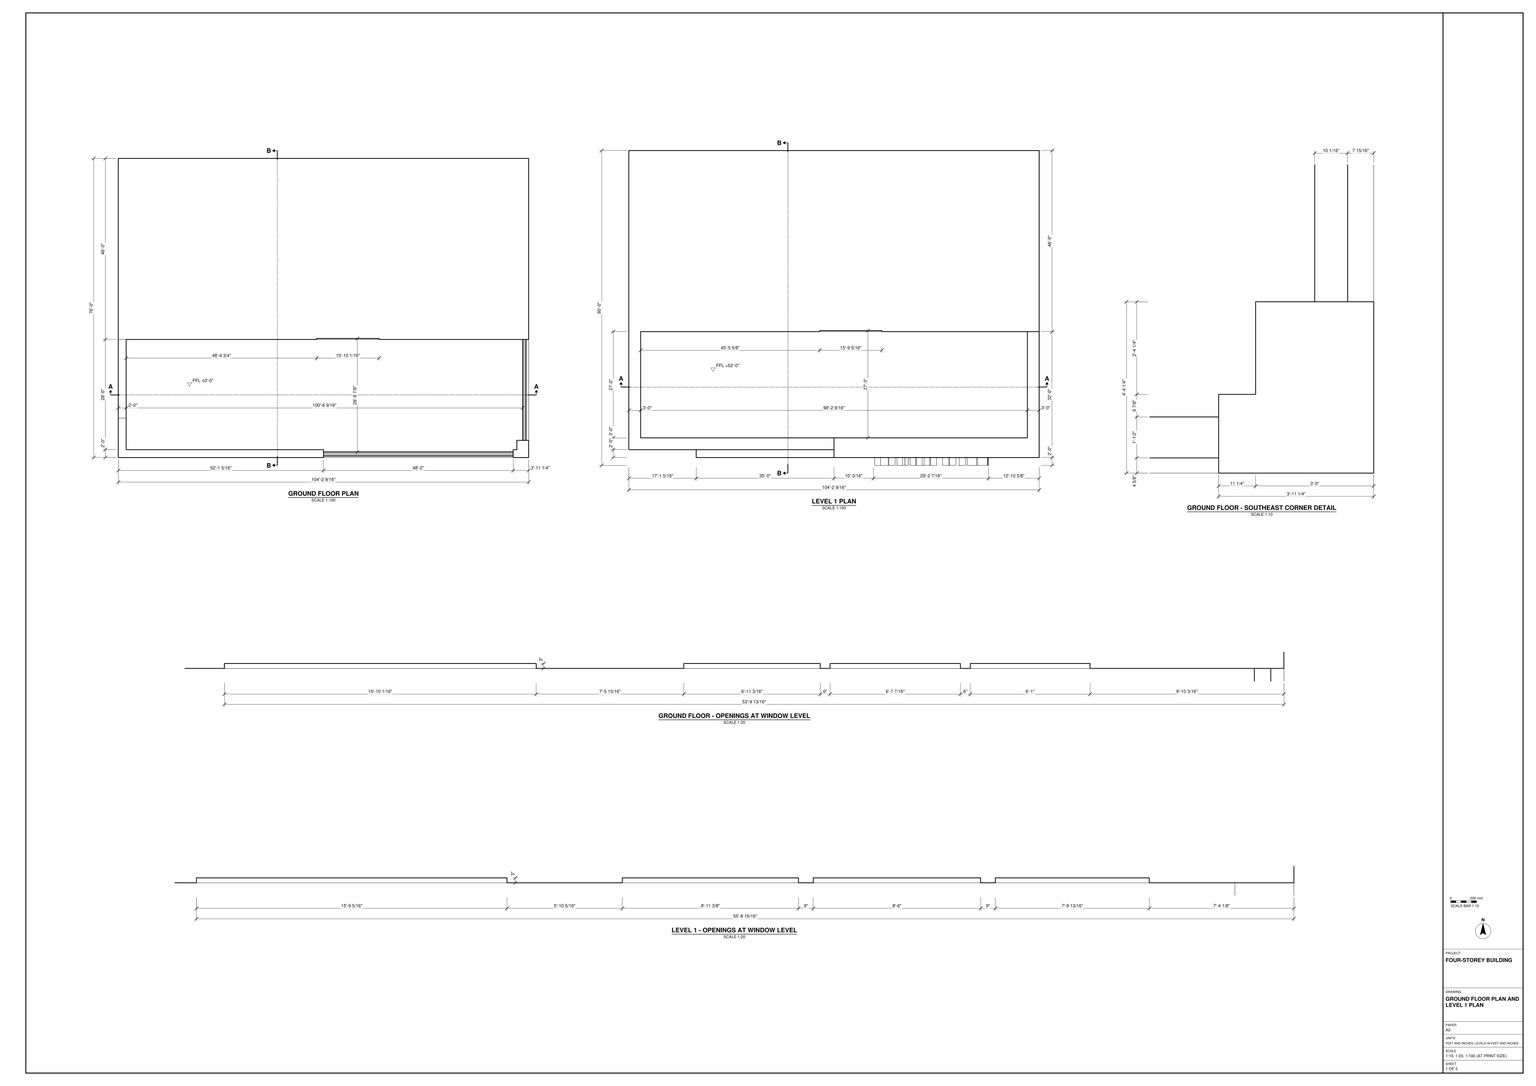
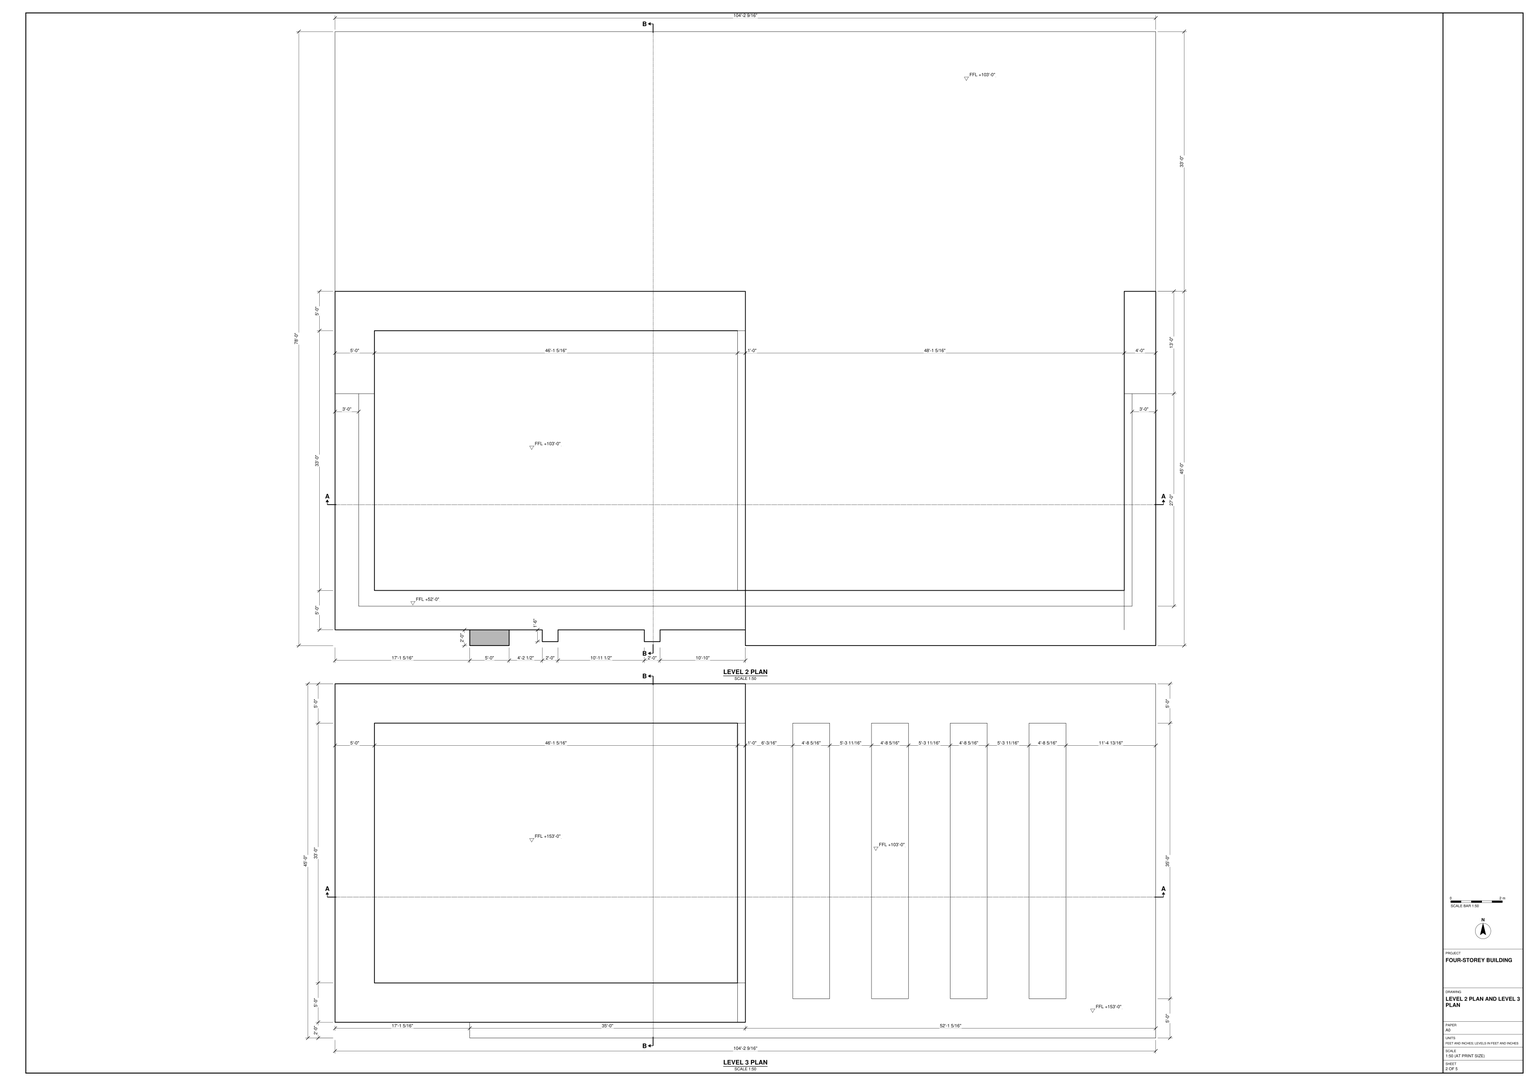
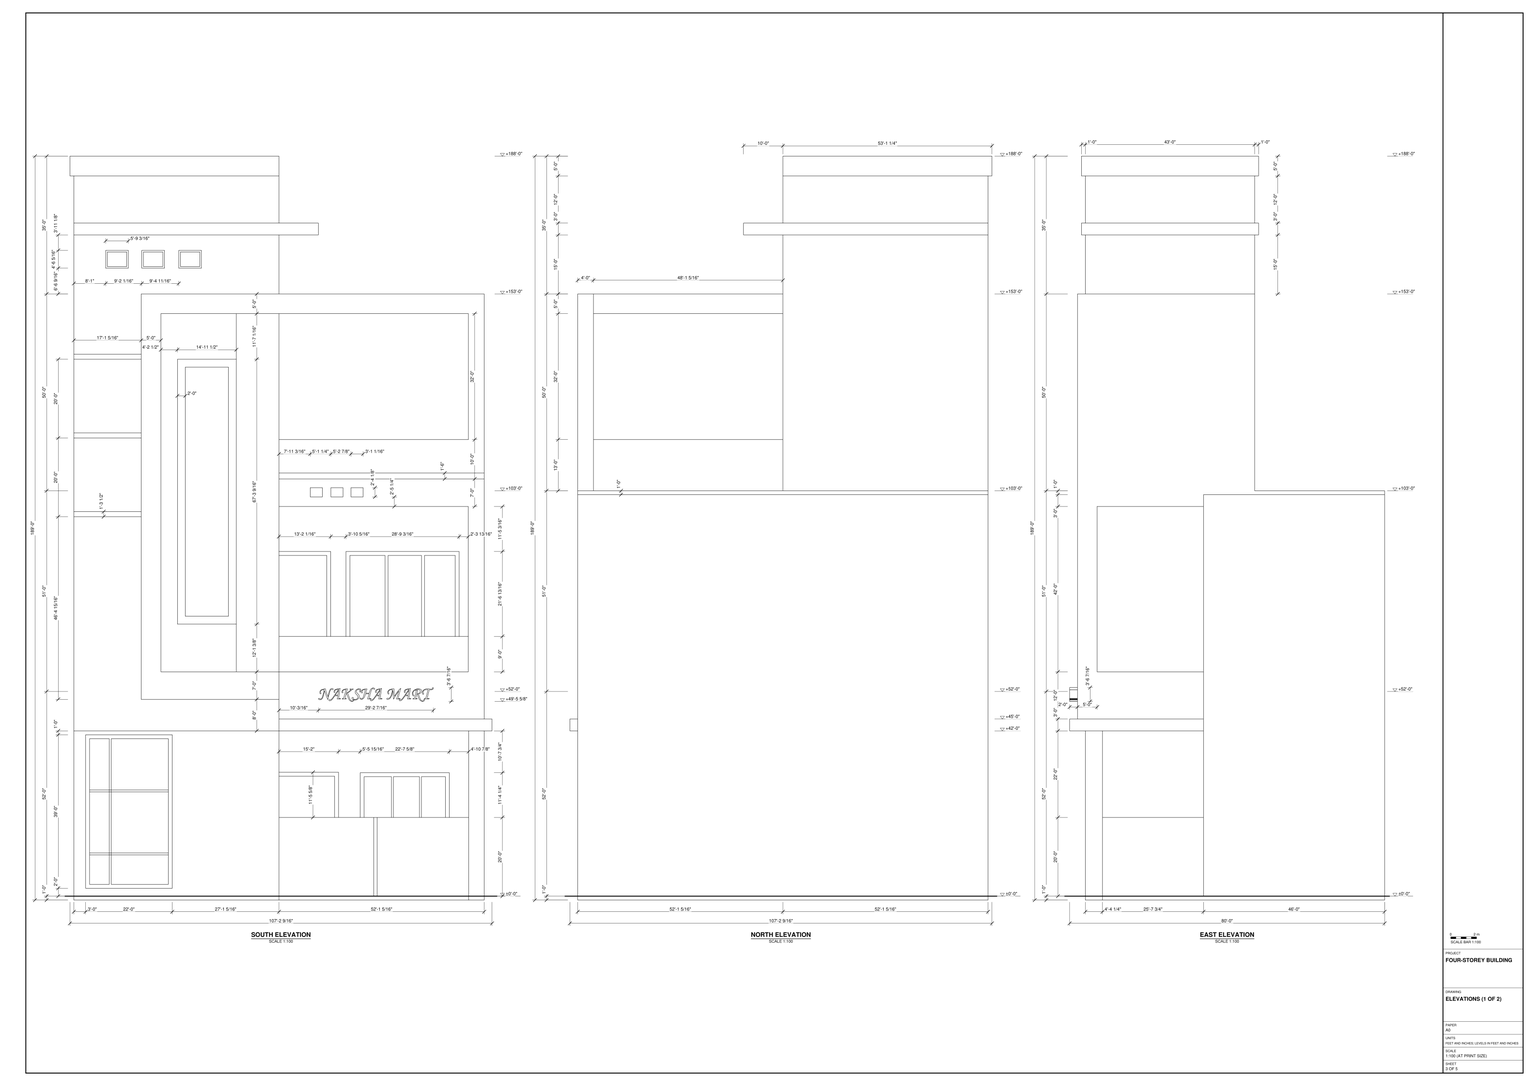
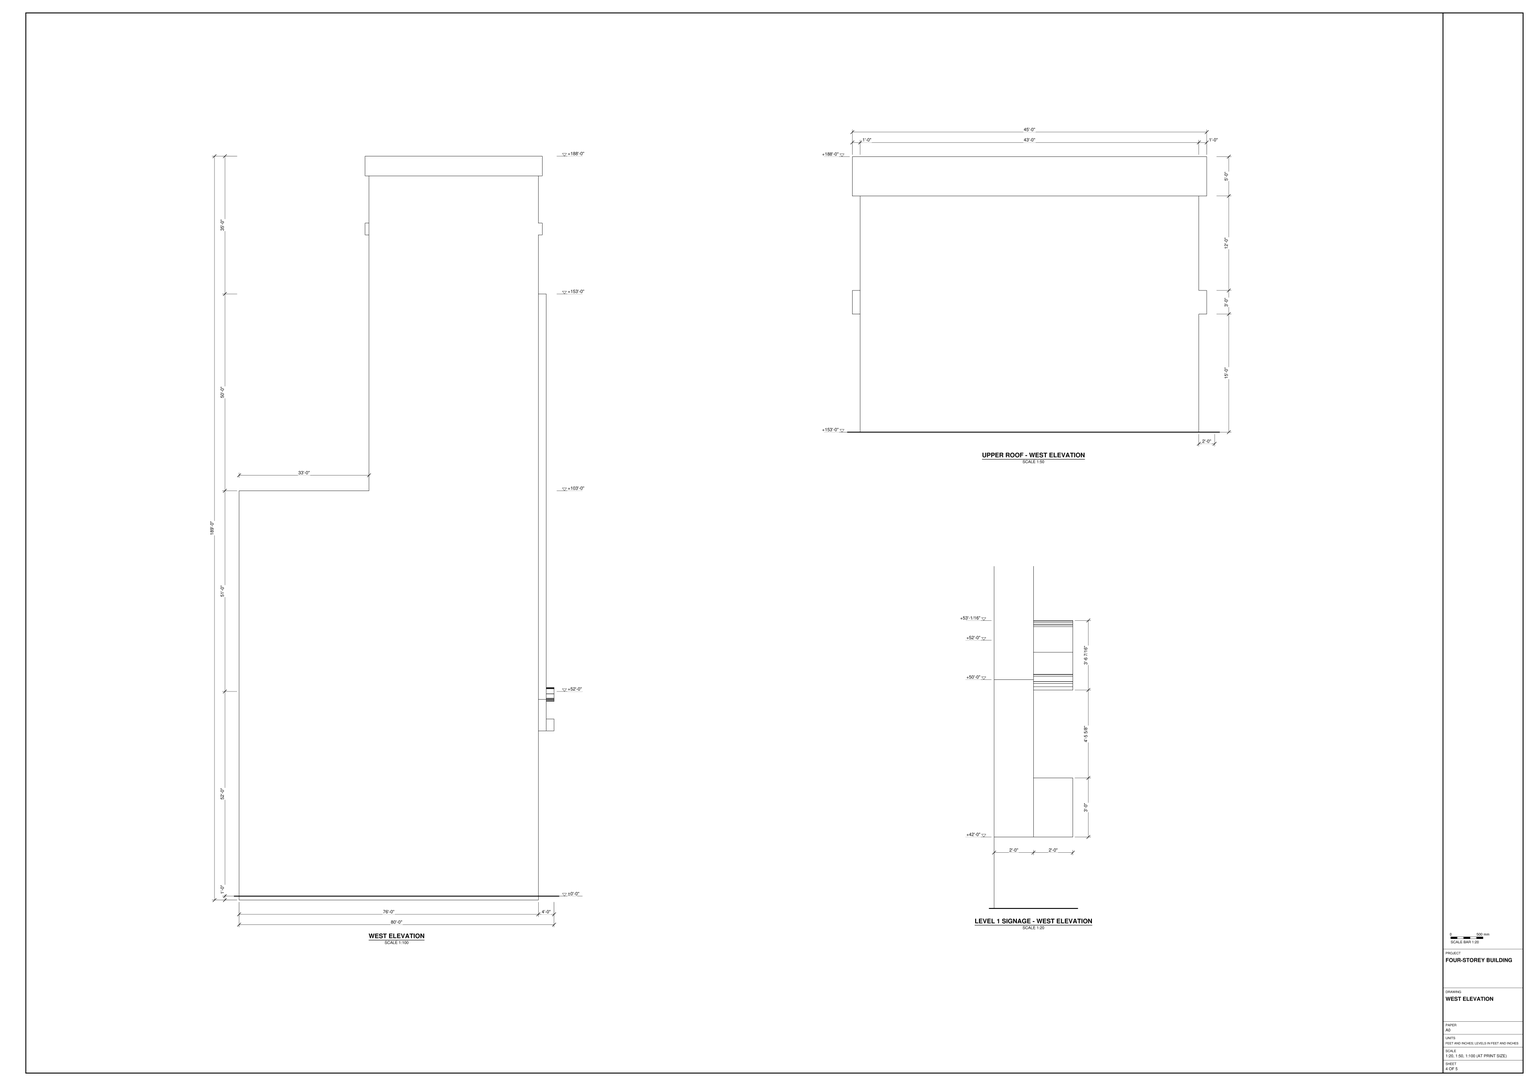
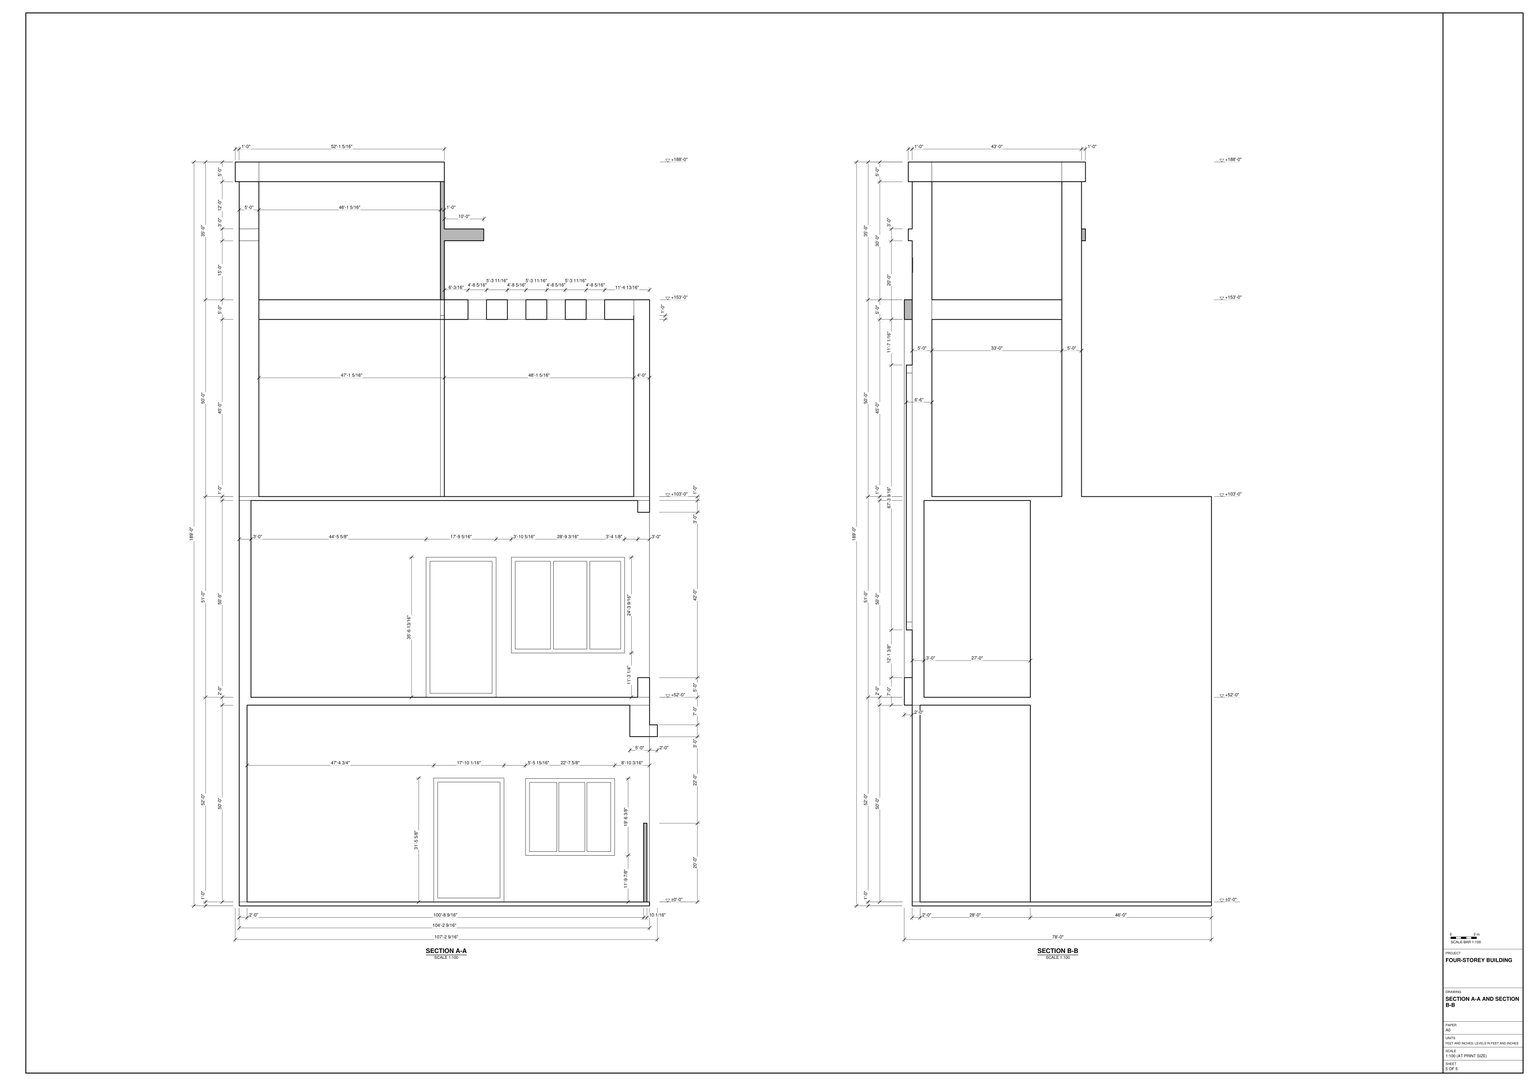
Build the four-storey building in SketchUp from task_files/diagram_01.pdf. Work in feet and inches. The overall dimensions, including projections, are 107'-2 9/16" east to west, 80'-0" north to south and 189'-0" high. Set the floor levels at ±0'-0", +52'-0", +103'-0" and +153'-0".

Use the plans to set out the wall thicknesses, slab edges and stepped southeast corner. Keep the broad lower roof at the rear, with the taller volumes towards the south. Above the east bay, form the long parallel openings shown in the upper slab so that the lower surface is visible through them. Carry the west bay up to its flat roof, distinguishing the roof cap from the projecting band below it.

Use the south elevation and window-level details to place the tall divided glazing on the west and the rows of openings on the east. Model the depth of the canopy, the large rectangular surround across the middle storeys and the tall inset panel within it. Keep walls, slabs and roof elements in separate groups or components, group each furniture or joinery piece shown separately, and use components for repeated parts. Decor and loose items, where shown, may be any suitable library components. Save one SketchUp model as output_files/four_storey_building_with_a_stepped_roofline.skp.

# SketchUp Ruby script. Lengths in inches.
U = 1.inch
M = Sketchup.active_model
def pt(a) = Geom::Point3d.new(a.map { |v| v * U })
def face(e, loops, mat)
  f = e.add_face(loops[0].map { |a| pt(a) })
  loops[1..].each { |l| e.add_face(l.map { |a| pt(a) }).erase! }
  f.material = f.back_material = mat if mat
  f
end
# faces: each face lists its corners as indices into pts; further lists are holes
def faces(e, pts, list, mat = nil) = list.each { |f| face(e, (f[0].is_a?(Array) ? f : [f]).map { |l| l.map { |i| pts[i] } }, mat) }
# xy, xz, yz: faces in a plane at the given z, y or x. An outline is a flat list of corners, or four numbers for a rectangle; further outlines are holes
def ring(l) = l.size == 4 ? [[l[0], l[1]], [l[2], l[1]], [l[2], l[3]], [l[0], l[3]]] : l.each_slice(2).to_a
def flat(e, list, mat, &to3) = list.each { |f| face(e, (f[0].is_a?(Array) ? f : [f]).map { |l| ring(l).map { |u, v| to3.(u, v) } }, mat) }
def xy(e, z, list, mat = nil) = flat(e, list, mat) { |x, y| [x, y, z] }
def xz(e, y, list, mat = nil) = flat(e, list, mat) { |x, z| [x, y, z] }
def yz(e, x, list, mat = nil) = flat(e, list, mat) { |y, z| [x, y, z] }
def lines(e, pts, list) = list.each { |a, b| e.add_line(pt(pts[a]), pt(pts[b])) }
# prism: a flat outline (further loops are holes) pulled along v
def prism(e, loops, v, mat = nil)
  f = face(e, loops, mat); d = Geom::Vector3d.new(v.map { |x| x * U })
  f.pushpull(f.normal.samedirection?(d) ? d.length : -d.length)
end
def box(e, o, s, mat = nil) = prism(e, [[o, [o[0] + s[0], o[1], o[2]], [o[0] + s[0], o[1] + s[1], o[2]], [o[0], o[1] + s[1], o[2]]]], [0, 0, s[2]], mat)
def at(x, y, z, deg = 0) = Geom::Transformation.translation(pt([x, y, z])) * Geom::Transformation.rotation(ORIGIN, Z_AXIS, deg.degrees)
def axes(o, x, y, z) = Geom::Transformation.new([*x, 0, *y, 0, *z, 0, *pt(o).to_a, 1])
def part(name) = M.definitions.add(name)
# library, detail: a bought-in or finely detailed component or shape, given as its bounding box
def library(name, o, s) = part(name).tap { |d| box(d.entities, o, s) }
def detail(e, o, s) = box(e.add_group.entities, o, s)
def put(e, d, t, mat = nil) = e.add_instance(d, t).tap { |i| i.material = mat if mat }
def group(e, t, mat = nil) = e.add_group.tap { |g| g.transformation = t; g.material = mat if mat }.entities
root = M.entities
M.materials.add("[0009_Linen]").color = [250, 240, 230]
M.materials.add("[0012_Bisque]").color = [211, 189, 162]
M.materials.add("[0012_Bisque]1").color = [191, 171, 147]
M.materials.add("[0012_Bisque]2").color = [211, 189, 162]
M.materials.add("[0022_Maroon]").color = [128, 0, 0]
M.materials.add("[0043_SaddleBrown]").color = [61, 30, 8]
M.materials.add("[0111_SlateGray]").color = [87, 99, 112]
M.materials.add("[0111_SlateGray]1").color = [97, 111, 124]
M.materials.add("[0135_DarkGray]").color = [43, 43, 43]
M.materials.add("[Granite Dark Gray]").color = [69, 68, 68]
M.materials.add("[Grass Dark Green]").color = [106, 157, 55]
M.materials.add("[Translucent Glass Gray]").color = [128, 121, 75]
M.materials["[Translucent Glass Gray]"].alpha = 0.5
M.materials.add("[Wood Veneer 01]").color = [120, 70, 37]
c1 = part("NAKSHA MART")
detail(c1.entities,[2.27,5.2,0],[45.06,34.4,24])
detail(c1.entities,[33.93,2.07,0],[35.8,38.06,24])
detail(c1.entities,[73.53,0,0],[57.92,38.5,24])
detail(c1.entities,[128.62,6.35,0],[45.23,34.91,24])
detail(c1.entities,[160.41,2.07,0],[35.79,38.06,24])
detail(c1.entities,[210.23,6.17,0],[43.05,33.86,24])
detail(c1.entities,[248.17,2.07,0],[35.8,38.06,24])
detail(c1.entities,[288.18,0.15,0],[37.66,38.48,24])
detail(c1.entities,[318.72,7.5,0],[34.01,34.93,24])
xy(root,0,[[12,48,1262.5625,168],[12,168,1262.5625,960]])
xy(root,12,[[637.28,52.64,1215.29,65.13],[1244.5625,100.24,1254.6,408],[12,408,1262.5625,960]])
xy(root,12,[[1254.6,100.24,1262.5625,408]],"[0012_Bisque]1")
xy(root,12,[[637.28,65.13,1215.29,65.13,1215.29,72,1226.5625,72,1226.5625,100.24,1244.5625,100.24,1244.5625,408,36,408,36,72,637.28,72]],"[Granite Dark Gray]")
xy(root,12,[[637.28,48,1215.29,52.64]],"[Wood Veneer 01]")
xy(root,24,[[616.77,408,806.84,411]])
xy(root,165.9,[[896.77,408,979.96,411],[985.96,408,1065.4,411],[1071.4,408,1144.39,411]])
xy(root,252,[[1244.5625,100.24,1254.6,408]],"[0012_Bisque]1")
xy(root,252,[[637.28,52.64,1215.29,65.13]],"[0022_Maroon]")
xy(root,376.27,[[896.77,408,979.96,411],[985.96,408,1065.4,411],[1071.4,408,1144.39,411]])
xy(root,377.625,[[616.77,408,806.84,411]])
xy(root,516,[[637.28,0,637.28,72,1202.5625,72,1202.5625,408,1262.5625,408,1262.5625,100.24,1226.5625,100.24,1226.5625,72,1215.29,72,1215.29,48,1262.5625,48,1262.5625,408,1286.5625,408,1286.5625,0]])
xy(root,552,[[637.28,0,1286.5625,0,1286.5625,408,1262.5625,408,1262.5625,24,637.28,24]])
xy(root,612,[[36,72,1202.5625,408]])
xy(root,612,[[217.28,24,637.28,48]],"[0012_Bisque]")
xy(root,636,[[48,84,1226.5625,408]],"[Grass Dark Green]")
xy(root,648,[[593.64,408,782.93,411]])
xy(root,696,[[277.28,24,637.28,48],[637.28,24,1214.24,54],[1226.5625,84,1262.5625,408]],"[0012_Bisque]")
xy(root,783.23,[[853.22,408,960.6,411],[969.6,408,1071.6,411],[1080.6,408,1174.41,411]])
xy(root,804,[[637.28,54,1214.24,84]],"[0111_SlateGray]1")
xy(root,841.35,[[327.77,30,507.27,48]])
xy(root,865.35,[[351.77,30,483.27,48]])
xy(root,1050.8,[[593.64,408,782.93,411],[853.22,408,960.6,411],[969.6,408,1071.6,411],[1080.6,408,1174.41,411]])
xy(root,1200,[[637.28,24,1214.24,84],[1226.5625,84,1262.5625,408]],"[0012_Bisque]")
xy(root,1236,[[48,84,1226.5625,408]],"[0012_Bisque]")
xy(root,1248,[[72,108,625.28,504],[625.28,108,637.28,504]])
xy(root,1248,[[637.28,108,1214.5625,108,1214.5625,564,1262.5625,564,1262.5625,960,12,960,12,564,637.28,564]],"[0009_Linen]")
xy(root,1404,[[637.28,24,1214.5625,108]])
xy(root,1624.92,[[351.77,30,483.27,48]])
xy(root,1648.92,[[327.77,30,507.27,48]])
xy(root,1788,[[625.28,48,637.28,108]])
xy(root,1788,[[[277.28,24,277.28,48,637.28,48,637.28,108,72,108,72,504,637.28,504,637.28,564,1214.5625,564,1214.5625,24],[829.44,84,885.76,504],[709.44,84,765.76,504],[1069.44,84,1125.76,504],[949.44,84,1005.76,504]]],"[0012_Bisque]")
xy(root,1848,[[625.28,48,637.28,108],[72,108,625.28,504],[625.28,108,637.28,504]])
xy(root,1848,[[[217.28,24,1262.5625,24,1262.5625,564,637.28,564,637.28,48,217.28,48],[829.44,84,885.76,504],[709.44,84,765.76,504],[1069.44,84,1125.76,504],[949.44,84,1005.76,504]]],"[0012_Bisque]")
xy(root,1931.55,[[114.01,48,173.2,50],[224.08,48,283.26,50],[336.76,48,395.95,50]])
xy(root,1975.86,[[114.01,48,173.2,50],[224.08,48,283.26,50],[336.76,48,395.95,50]])
xy(root,2028,[[702.53,79.04,699.42,79.45,696.53,80.65,694.04,82.56,692.14,85.04,690.9375,87.9375,690.53,91.04,690.9375,94.15,692.14,97.04,694.04,99.53,696.53,101.4375,699.42,102.64,702.53,103.04,705.63,102.64,708.53,101.4375,711.01,99.53,712.92,97.04,714.12,94.15,714.53,91.04,714.12,87.9375,712.92,85.04,711.01,82.56,708.53,80.65,705.63,79.45],[702.53,208.98,699.42,209.39,696.53,210.59,694.04,212.5,692.14,214.98,690.9375,217.875,690.53,220.98,690.9375,224.09,692.14,226.98,694.04,229.47,696.53,231.375,699.42,232.57,702.53,232.98,705.63,232.57,708.53,231.375,711.01,229.47,712.92,226.98,714.12,224.09,714.53,220.98,714.12,217.875,712.92,214.98,711.01,212.5,708.53,210.59,705.63,209.39],[702.53,430.29,699.42,430.7,696.53,431.9,694.04,433.81,692.14,436.29,690.9375,439.1875,690.53,442.29,690.9375,445.4,692.14,448.29,694.04,450.78,696.53,452.6875,699.42,453.89,702.53,454.29,705.63,453.89,708.53,452.6875,711.01,450.78,712.92,448.29,714.12,445.4,714.53,442.29,714.12,439.1875,712.92,436.29,711.01,433.81,708.53,431.9,705.63,430.7]])
xy(root,2028,[[[12,36,12,48,637.28,48,637.28,564,12,564,12,576,757.28,576,757.28,36],[702.53,79.04,705.63,79.45,708.53,80.65,711.01,82.56,712.92,85.04,714.12,87.9375,714.53,91.04,714.12,94.15,712.92,97.04,711.01,99.53,708.53,101.4375,705.63,102.64,702.53,103.04,699.42,102.64,696.53,101.4375,694.04,99.53,692.14,97.04,690.9375,94.15,690.53,91.04,690.9375,87.9375,692.14,85.04,694.04,82.56,696.53,80.65,699.42,79.45],[702.53,430.29,705.63,430.7,708.53,431.9,711.01,433.81,712.92,436.29,714.12,439.1875,714.53,442.29,714.12,445.4,712.92,448.29,711.01,450.78,708.53,452.6875,705.63,453.89,702.53,454.29,699.42,453.89,696.53,452.6875,694.04,450.78,692.14,448.29,690.9375,445.4,690.53,442.29,690.9375,439.1875,692.14,436.29,694.04,433.81,696.53,431.9,699.42,430.7],[702.53,208.98,705.63,209.39,708.53,210.59,711.01,212.5,712.92,214.98,714.12,217.875,714.53,220.98,714.12,224.09,712.92,226.98,711.01,229.47,708.53,231.375,705.63,232.57,702.53,232.98,699.42,232.57,696.53,231.375,694.04,229.47,692.14,226.98,690.9375,224.09,690.53,220.98,690.9375,217.875,692.14,214.98,694.04,212.5,696.53,210.59,699.42,209.39]]],"[0012_Bisque]")
xy(root,2064,[[12,36,757.28,36,757.28,576,12,576,12,564,637.28,564,637.28,48,12,48]],"[0012_Bisque]")
xy(root,2208,[[12,48,12,564,637.28,564,637.28,504,72,504,72,108,637.28,108,637.28,48],[72,108,625.28,504],[625.28,108,637.28,504]])
xy(root,2208,[[0,36,0,576,637.28,576,637.28,564,12,564,12,48,637.28,48,637.28,36]],"[0012_Bisque]")
xy(root,2268,[[0,36,637.28,576]],"[0012_Bisque]")
xz(root,0,[[637.28,516,1286.5625,552]])
xz(root,24,[[637.28,1284,1262.5625,1302]])
xz(root,24,[[[637.28,552,1262.5625,552,1262.5625,1284,637.28,1284,637.28,1200,1214.24,1200,1214.24,696,637.28,696],[732.45,1229.22,769.52,1257.35],[795.33,1229.22,832.39,1257.35],[856.58,1229.22,893.64,1257.35]],[217.28,612,637.28,612,637.28,696,277.28,696,277.28,1788,1214.5625,1788,1214.5625,1404,637.28,1404,637.28,1302,1262.5625,1302,1262.5625,1848,217.28,1848]],"[0012_Bisque]")
xz(root,24,[[732.45,1229.22,769.52,1257.35],[795.33,1229.22,832.39,1257.35],[856.58,1229.22,893.64,1257.35]],"[0135_DarkGray]")
xz(root,30,[[[327.77,841.35,507.27,1648.92],[351.77,865.35,483.27,1624.92]]])
xz(root,36,[[12,2028,757.28,2064],[0,2208,637.28,2268]],"[0012_Bisque]")
xz(root,48,[[1215.29,0,1262.5625,516],[217.28,612,217.28,1848,637.28,1848,637.28,1788,277.28,1788,277.28,696,637.28,696,637.28,612],[12,1168.92,217.28,1184.41],[12,1408.92,217.28,1424.41],[12,1648.92,217.28,1664.41],
  [[109.01,1926.55,178.2,1980.86],[114.01,1931.55,173.2,1975.86]],[[219.08,1926.55,288.26,1980.86],[224.08,1931.55,283.26,1975.86]],[[331.76,1926.55,400.95,1980.86],[336.76,1931.55,395.95,1975.86]]])
xz(root,48,[[[12,0,637.28,516],[48,36,312,504]]],"[0012_Bisque]2")
xz(root,48,[[12,516,637.28,516,637.28,612,217.28,612,217.28,1168.92,12,1168.92],[12,1184.41,217.28,1408.92],[12,1424.41,217.28,1648.92],[[12,1664.41,217.28,1664.41,217.28,1848,637.28,1848,637.28,2028,12,2028],[331.76,1926.55,400.95,1980.86],[219.08,1926.55,288.26,1980.86],[109.01,1926.55,178.2,1980.86]],[12,2064,637.28,2208]],"[0111_SlateGray]")
xz(root,48,[[277.28,696,507.27,696,507.27,841.35,327.77,841.35,327.77,1648.92,507.27,1648.92,507.27,1788,277.28,1788]],"[0135_DarkGray]")
xz(root,48,[[351.77,865.35,483.27,1624.92]],"[Translucent Glass Gray]")
xz(root,48,[[637.28,0,1215.29,12],[[48,36,312,504],[60,48,60,492,120,492,120,336,126,336,126,492,300,492,300,48,126,48,126,138,120,138,120,48]],[60,48,120,138],[126,48,300,138],[60,138,120,144],
  [120,138,126,144],[126,138,300,144],[60,144,120,330],[120,144,126,330],[126,144,300,330],
  [60,330,120,336],[120,330,126,336],[126,330,300,336],[60,336,120,492],[126,336,300,492],
  [507.27,696,637.28,1788]],"[Wood Veneer 01]")
xz(root,50,[[114.01,1931.55,173.2,1975.86],[224.08,1931.55,283.26,1975.86],[336.76,1931.55,395.95,1975.86]])
xz(root,52.64,[[637.28,12,926.29,252],[926.29,12,936.34,252],[936.34,12,1215.29,252]],"[Wood Veneer 01]")
xz(root,54,[[637.28,696,1214.24,804]],"[0111_SlateGray]1")
xz(root,65.13,[[637.28,12,1215.29,252]],"[0022_Maroon]")
xz(root,72,[[1215.29,12,1226.5625,516],[637.28,516,1202.5625,612]])
xz(root,72,[[36,12,637.28,612]],"[0012_Bisque]1")
xz(root,84,[[709.44,1788,765.76,1848],[829.44,1788,885.76,1848],[949.44,1788,1005.76,1848],[1069.44,1788,1125.76,1848]])
xz(root,84,[[48,636,637.28,1236],[1214.24,696,1226.5625,1200],[1226.5625,696,1262.5625,1200],[637.28,1200,1226.5625,1236]],"[0012_Bisque]")
xz(root,84,[[637.28,636,637.28,804,1214.24,804,1214.24,696,1226.5625,696,1226.5625,636]],"[0111_SlateGray]1")
xz(root,100.24,[[1226.5625,12,1226.5625,516,1262.5625,516,1262.5625,12,1254.6,12,1254.6,252,1244.5625,252,1244.5625,12],[1244.5625,12,1254.6,252]])
xz(root,108,[[72,1248,625.28,1788],[625.28,1248,637.28,1404],[637.28,1248,1214.5625,1404],[72,1848,625.28,2208]])
xz(root,408,[[1244.5625,12,1254.6,252],[1202.5625,516,1262.5625,612],[1262.5625,516,1286.5625,552],[1226.5625,636,1262.5625,696],[1226.5625,1200,1262.5625,1236]])
xz(root,408,[[[48,636,581.64,636,581.64,1062.8,794.93,1062.8,794.93,636,1226.5625,636,1226.5625,696,1262.5625,696,1262.5625,1200,1226.5625,1200,1226.5625,1236,48,1236],[841.22,771.23,1186.41,1062.8]]],"[0012_Bisque]")
xz(root,408,[[[36,12,604.77,12,604.77,389.625,818.84,389.625,818.84,12,1244.5625,12,1244.5625,252,1254.6,252,1254.6,12,1262.5625,12,1262.5625,516,1202.5625,516,1202.5625,612,36,612],[884.77,153.9,1156.39,388.27]]],"[0012_Bisque]1")
xz(root,408,[[[604.77,12,818.84,389.625],[616.77,24,806.84,377.625]],[[884.77,153.9,1156.39,388.27],[896.77,165.9,979.96,376.27],[985.96,165.9,1065.4,376.27],[1071.4,165.9,1144.39,376.27]],[[581.64,636,794.93,1062.8],[593.64,648,782.93,1050.8]],[[841.22,771.23,1186.41,1062.8],[853.22,783.23,960.6,1050.8],[969.6,783.23,1071.6,1050.8],[1080.6,783.23,1174.41,1050.8]]],"[0043_SaddleBrown]")
xz(root,411,[[616.77,24,806.84,377.625],[593.64,648,782.93,1050.8]],"[0043_SaddleBrown]")
xz(root,411,[[896.77,165.9,979.96,376.27],[985.96,165.9,1065.4,376.27],[1071.4,165.9,1144.39,376.27],[853.22,783.23,960.6,1050.8],[969.6,783.23,1071.6,1050.8],
  [1080.6,783.23,1174.41,1050.8]],"[Translucent Glass Gray]")
xz(root,504,[[72,1248,625.28,1788],[72,1788,625.28,1848],[625.28,1788,637.28,1800],[709.44,1788,765.76,1848],[829.44,1788,885.76,1848],
  [949.44,1788,1005.76,1848],[1069.44,1788,1125.76,1848],[625.28,1800,637.28,1848],[72,1848,625.28,2208]])
xz(root,564,[[1214.5625,1248,1262.5625,1848],[637.28,1788,1214.5625,1848],[12,2028,637.28,2064]])
xz(root,564,[[12,1248,637.28,2028],[12,2064,637.28,2208]],"[0135_DarkGray]")
xz(root,576,[[12,2028,757.28,2064]])
xz(root,576,[[0,2208,637.28,2268]],"[0012_Bisque]")
xz(root,960,[[12,0,1262.5625,12],[12,1236,1262.5625,1248]])
xz(root,960,[[12,12,1262.5625,1236]],"[0009_Linen]")
yz(root,0,[[36,2208,576,2268]],"[0012_Bisque]")
yz(root,12,[[48,0,960,12],[564,2028,576,2064]])
yz(root,12,[[48,12,48,2028,36,2028,36,2064,48,2064,48,2208,564,2208,564,1248,960,1248,960,12]],"[0009_Linen]")
yz(root,36,[[72,12,408,612]],"[0012_Bisque]1")
yz(root,48,[[84,636,408,1236]],"[0012_Bisque]")
yz(root,72,[[108,1248,504,1788],[108,1788,504,1848],[108,1848,504,2208]])
yz(root,114.01,[[48,1931.55,50,1975.86]])
yz(root,173.2,[[48,1931.55,50,1975.86]])
yz(root,217.28,[[24,612,48,1848]],"[0012_Bisque]")
yz(root,224.08,[[48,1931.55,50,1975.86]])
yz(root,277.28,[[24,696,48,1788]],"[0012_Bisque]")
yz(root,283.26,[[48,1931.55,50,1975.86]])
yz(root,327.77,[[30,841.35,48,1648.92]])
yz(root,336.76,[[48,1931.55,50,1975.86]])
yz(root,351.77,[[30,865.35,48,1624.92]])
yz(root,395.95,[[48,1931.55,50,1975.86]])
yz(root,483.27,[[30,865.35,48,1624.92]])
yz(root,507.27,[[30,841.35,48,1648.92]])
yz(root,593.64,[[408,648,411,1050.8]])
yz(root,616.77,[[408,24,411,377.625]])
yz(root,625.28,[[108,1848,504,2208]])
yz(root,637.28,[[52.64,12,65.13,252],[48,516,72,612],[24,612,48,636],[24,636,48,696],[48,636,84,636,84,804,54,804,54,696,48,696],
  [24,1200,48,1404],[48,1200,84,1236],[48,1248,108,1404]])
yz(root,637.28,[[0,516,24,552],[24,516,48,612],[48,696,54,696,54,804,84,804,84,1200,48,1200],[36,2208,576,2268]],"[0012_Bisque]")
yz(root,637.28,[[48,12,52.64,12,52.64,252,65.13,252,65.13,12,72,12,72,516,48,516]],"[0012_Bisque]1")
yz(root,637.28,[[48,1848,564,2028],[48,2064,564,2208]],"[0111_SlateGray]")
yz(root,637.28,[[108,1248,564,1248,564,1788,504,1788,504,1848,48,1848,48,1404,108,1404]],"[0135_DarkGray]")
yz(root,709.44,[[84,1788,504,1848]])
yz(root,757.28,[[36,2028,576,2064]],"[0012_Bisque]")
yz(root,765.76,[[84,1788,504,1848]])
yz(root,782.93,[[408,648,411,1050.8]])
yz(root,806.84,[[408,24,411,377.625]])
yz(root,829.44,[[84,1788,504,1848]])
yz(root,853.22,[[408,783.23,411,1050.8]])
yz(root,885.76,[[84,1788,504,1848]])
yz(root,896.77,[[408,165.9,411,376.27]])
yz(root,949.44,[[84,1788,504,1848]])
yz(root,960.6,[[408,783.23,411,1050.8]])
yz(root,969.6,[[408,783.23,411,1050.8]])
yz(root,979.96,[[408,165.9,411,376.27]])
yz(root,985.96,[[408,165.9,411,376.27]])
yz(root,1005.76,[[84,1788,504,1848]])
yz(root,1065.4,[[408,165.9,411,376.27]])
yz(root,1069.44,[[84,1788,504,1848]])
yz(root,1071.4,[[408,165.9,411,376.27]])
yz(root,1071.6,[[408,783.23,411,1050.8]])
yz(root,1080.6,[[408,783.23,411,1050.8]])
yz(root,1125.76,[[84,1788,504,1848]])
yz(root,1144.39,[[408,165.9,411,376.27]])
yz(root,1174.41,[[408,783.23,411,1050.8]])
yz(root,1202.5625,[[72,516,408,612]])
yz(root,1214.24,[[24,696,24,1200,84,1200,84,804,54,804,54,696]],"[0012_Bisque]")
yz(root,1214.5625,[[108,1788,504,1800]])
yz(root,1214.5625,[[108,1248,108,1404,24,1404,24,1788,564,1788,564,1248]],"[0012_Bisque]")
yz(root,1215.29,[[48,12,48,516,72,516,72,12,65.13,12,65.13,252,52.64,252,52.64,12],[52.64,12,65.13,252]])
yz(root,1226.5625,[[72,12,100.24,516]])
yz(root,1226.5625,[[84,636,408,696],[84,1200,408,1236]],"[0012_Bisque]")
yz(root,1244.5625,[[100.24,12,408,252]],"[0012_Bisque]1")
yz(root,1254.6,[[100.24,12,408,252]],"[0012_Bisque]1")
yz(root,1262.5625,[[48,0,100.24,516]])
yz(root,1262.5625,[[408,12,960,1236]],"[0009_Linen]")
yz(root,1262.5625,[[24,552,408,552,408,696,84,696,84,1200,408,1200,408,1236,960,1236,960,1248,564,1248,564,1848,24,1848]],"[0012_Bisque]")
yz(root,1262.5625,[[100.24,0,960,12]],"[0012_Bisque]1")
yz(root,1286.5625,[[0,516,408,552]])
p = [[36,72,612],[36,48,612],[48,408,1236],[12,408,1236],[1214.5625,108,1248],[1214.5625,48,1248],
  [1214.5625,108,1800],[1214.5625,48,1800],[72,108,2208],[72,108,2268],[72,504,2208],[72,504,2268],
  [1262.5625,24,516],[1262.5625,24,552]]
lines(root,p,[[0,1],[2,3],[4,5],[6,7],[8,9],[10,11],[12,13]])
put(root,c1,axes([755.22,24,605.61],[1,0,0],[0,0,1],[0,-1,0]))
